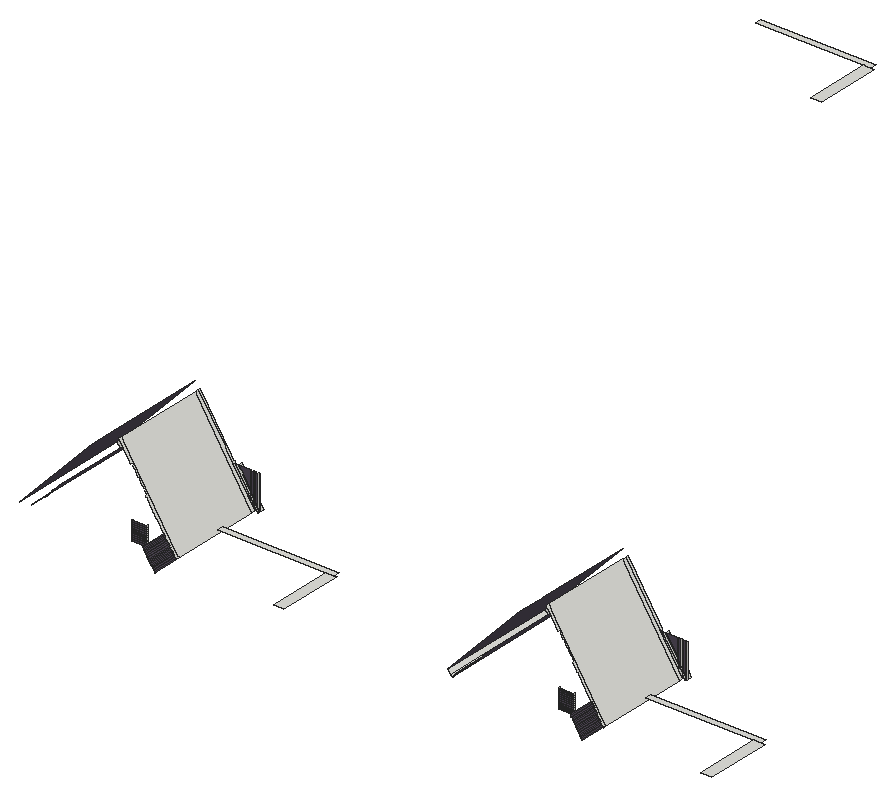
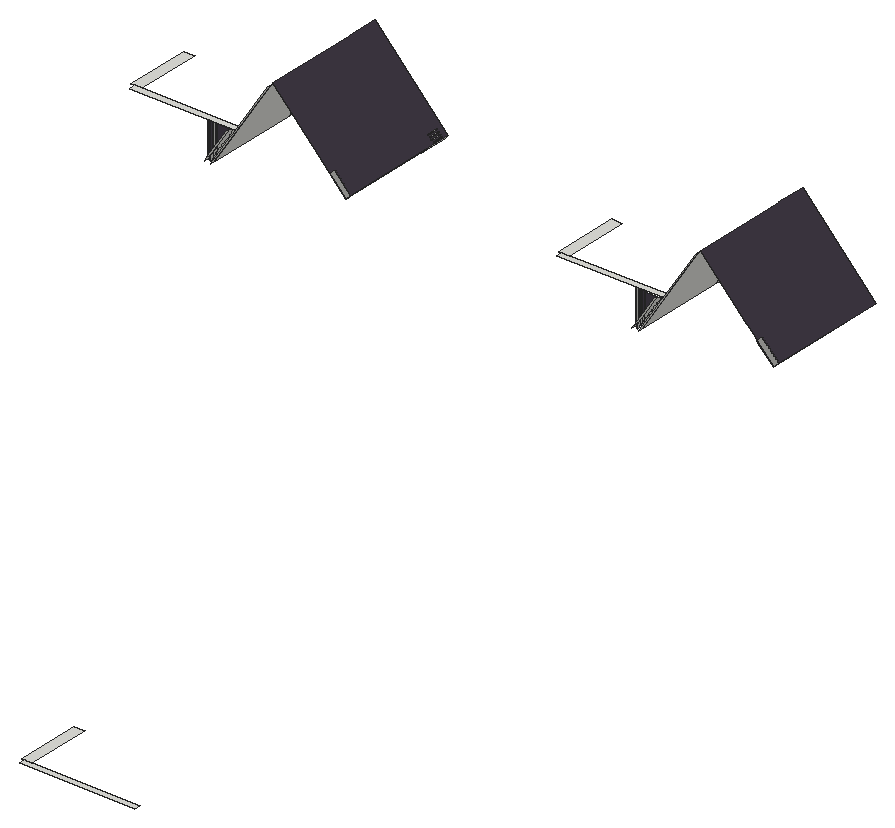
# SketchUp Ruby script. Lengths in inches.
U = 1.inch
M = Sketchup.active_model
def pt(a) = Geom::Point3d.new(a.map { |v| v * U })
def face(e, loops, mat)
  f = e.add_face(loops[0].map { |a| pt(a) })
  loops[1..].each { |l| e.add_face(l.map { |a| pt(a) }).erase! }
  f.material = f.back_material = mat if mat
  f
end
# faces: each face lists its corners as indices into pts; further lists are holes
def faces(e, pts, list, mat = nil) = list.each { |f| face(e, (f[0].is_a?(Array) ? f : [f]).map { |l| l.map { |i| pts[i] } }, mat) }
# xy, xz, yz: faces in a plane at the given z, y or x. An outline is a flat list of corners, or four numbers for a rectangle; further outlines are holes
def ring(l) = l.size == 4 ? [[l[0], l[1]], [l[2], l[1]], [l[2], l[3]], [l[0], l[3]]] : l.each_slice(2).to_a
def flat(e, list, mat, &to3) = list.each { |f| face(e, (f[0].is_a?(Array) ? f : [f]).map { |l| ring(l).map { |u, v| to3.(u, v) } }, mat) }
def xy(e, z, list, mat = nil) = flat(e, list, mat) { |x, y| [x, y, z] }
def xz(e, y, list, mat = nil) = flat(e, list, mat) { |x, z| [x, y, z] }
def yz(e, x, list, mat = nil) = flat(e, list, mat) { |y, z| [x, y, z] }
def lines(e, pts, list) = list.each { |a, b| e.add_line(pt(pts[a]), pt(pts[b])) }
# prism: a flat outline (further loops are holes) pulled along v
def prism(e, loops, v, mat = nil)
  f = face(e, loops, mat); d = Geom::Vector3d.new(v.map { |x| x * U })
  f.pushpull(f.normal.samedirection?(d) ? d.length : -d.length)
end
def box(e, o, s, mat = nil) = prism(e, [[o, [o[0] + s[0], o[1], o[2]], [o[0] + s[0], o[1] + s[1], o[2]], [o[0], o[1] + s[1], o[2]]]], [0, 0, s[2]], mat)
def at(x, y, z, deg = 0) = Geom::Transformation.translation(pt([x, y, z])) * Geom::Transformation.rotation(ORIGIN, Z_AXIS, deg.degrees)
def axes(o, x, y, z) = Geom::Transformation.new([*x, 0, *y, 0, *z, 0, *pt(o).to_a, 1])
def part(name) = M.definitions.add(name)
# library, detail: a bought-in or finely detailed component or shape, given as its bounding box
def library(name, o, s) = part(name).tap { |d| box(d.entities, o, s) }
def detail(e, o, s) = box(e.add_group.entities, o, s)
def put(e, d, t, mat = nil) = e.add_instance(d, t).tap { |i| i.material = mat if mat }
def group(e, t, mat = nil) = e.add_group.tap { |g| g.transformation = t; g.material = mat if mat }.entities
root = M.entities
M.materials.add("[Color M06]").color = [79, 71, 84]
xy(root,267.02,[[1464.52,523.75,1495.49,526.125],[2350.98,523.75,2381.95,526.125]])
xy(root,267.83,[[1464.52,523.75,1495.49,526.125],[2350.98,523.75,2381.95,526.125]])
xy(root,270.95,[[1464.52,523.75,1495.49,526.125],[2350.98,523.75,2381.95,526.125]])
xy(root,271.76,[[1464.52,523.75,1495.49,526.125],[2350.98,523.75,2381.95,526.125]])
xy(root,274.89,[[1464.52,523.75,1495.49,526.125],[2350.98,523.75,2381.95,526.125]])
xy(root,275.7,[[1464.52,523.75,1495.49,526.125],[2350.98,523.75,2381.95,526.125]])
xy(root,278.1875,[[1787.6875,487.3125,1810.23,623.84],[2674.15,487.3125,2696.7,623.84],[1563.99,623.84,1803.23,636.82],[2450.46,623.84,2689.7,636.82],[1419.96,2339.31,1442.5,2475.84],
  [1196.26,2475.84,1435.5,2488.81]])
xy(root,278.83,[[1464.52,523.75,1495.49,526.125],[2350.98,523.75,2381.95,526.125]])
xy(root,279.64,[[1464.52,523.75,1495.49,526.125],[2350.98,523.75,2381.95,526.125]])
xy(root,282.77,[[1464.52,523.75,1495.49,526.125],[2350.98,523.75,2381.95,526.125]])
xy(root,283.58,[[1464.52,523.75,1495.49,526.125],[2350.98,523.75,2381.95,526.125]],"[Color M06]")
xy(root,286.7,[[1464.52,523.75,1495.49,526.125],[2350.98,523.75,2381.95,526.125]])
xy(root,287.51,[[1464.52,523.75,1495.49,526.125],[2350.98,523.75,2381.95,526.125]],"[Color M06]")
xy(root,290.64,[[1464.52,523.75,1495.49,526.125],[2350.98,523.75,2381.95,526.125]])
xy(root,291.45,[[1464.52,523.75,1495.49,526.125],[2350.98,523.75,2381.95,526.125]],"[Color M06]")
xy(root,294.58,[[1464.52,523.75,1495.49,526.125],[2350.98,523.75,2381.95,526.125]])
xy(root,295.39,[[1464.52,523.75,1495.49,526.125],[2350.98,523.75,2381.95,526.125]])
xy(root,298.52,[[1464.52,523.75,1495.49,526.125],[2350.98,523.75,2381.95,526.125]])
xy(root,299.33,[[1464.52,523.75,1495.49,526.125],[2350.98,523.75,2381.95,526.125]])
xy(root,302.45,[[1464.52,523.75,1495.49,526.125],[2350.98,523.75,2381.95,526.125]])
xy(root,303.26,[[1464.52,523.75,1495.49,526.125],[2350.98,523.75,2381.95,526.125]])
xz(root,521.5625,[[1557.92,265.95,1557.66,266.36,1557.92,266.53],[2444.39,265.95,2444.125,266.36,2444.39,266.53],[1557.13,267.19,1557.39,267.36,1555.7,270,1555.43,269.84],[2443.59,267.19,2443.86,267.36,2442.16,270,2441.9,269.84],[1554.9,270.67,1555.16,270.83,1553.47,273.48,1553.21,273.31],
  [2441.37,270.67,2441.63,270.83,2439.93,273.48,2439.67,273.31],[1552.68,274.14,1552.9375,274.31,1551.24,276.95,1550.98,276.78],[2439.14,274.14,2439.4,274.31,2437.71,276.95,2437.44,276.78],[1550.45,277.61,1550.71,277.78,1549.02,280.42,1548.75,280.25],[2436.91,277.61,2437.18,277.78,2435.48,280.42,2435.22,280.25],
  [1548.22,281.08,1548.49,281.25,1546.79,283.89,1546.53,283.73],[2434.6875,281.08,2434.95,281.25,2433.26,283.89,2432.99,283.73],[1546,284.56,1546.26,284.72,1544.56,287.37,1544.3,287.2],[2432.46,284.56,2432.72,284.72,2431.03,287.37,2430.77,287.2],[1543.77,288.03,1544.03,288.2,1542.34,290.84,1542.08,290.67],
  [2430.23,288.03,2430.5,288.2,2428.8,290.84,2428.54,290.67],[1289.04,289.13,1288.59,289.56,1291.01,292.13,1291.46,291.7],[2175.5,289.13,2175.05,289.56,2177.47,292.13,2177.93,291.7],[1541.54,291.5,1539.85,294.14,1540.11,294.3125,1541.81,291.67],[1541.54,291.5,1541.81,291.67,1540.11,294.3125,1539.85,294.14],
  [2428.01,291.5,2426.3125,294.14,2426.58,294.3125,2428.27,291.67],[1292.34,292.64,1291.88,293.0625,1294.3,295.64,1294.76,295.21],[2178.8,292.64,2178.35,293.0625,2180.77,295.64,2181.22,295.21],[1539.32,294.97,1537.62,297.62,1537.89,297.79,1539.58,295.14],[2425.78,294.97,2426.04,295.14,2424.35,297.79,2424.09,297.62],
  [1295.64,296.14,1295.18,296.57,1297.6,299.14,1298.06,298.71],[2182.1,296.14,2181.65,296.57,2184.07,299.14,2184.52,298.71],[1537.09,298.45,1535.4,301.09,1535.66,301.26,1537.35,298.61],[2423.55,298.45,2423.82,298.61,2422.125,301.26,2421.86,301.09],[1298.9375,299.64,1298.48,300.07,1300.9,302.64,1301.36,302.22],
  [2185.4,299.64,2184.94,300.07,2187.37,302.64,2187.82,302.22],[1534.76,301.85,1535.13,302.09,1533.43,304.73,1533.07,304.49],[2421.22,301.85,2421.59,302.09,2419.9,304.73,2419.53,304.49],[1302.23,303.15,1301.78,303.58,1304.2,306.15,1304.66,305.72],[2188.7,303.15,2188.24,303.58,2190.66,306.15,2191.12,305.72],
  [1301.78,303.58,1301.55,303.79,1303.97,306.36,1304.2,306.15],[2188.24,303.58,2188.02,303.79,2190.4375,306.36,2190.66,306.15]])
xz(root,523.75,[[1464.52,267.83,1495.49,270.95],[2350.98,267.83,2381.95,270.95],[1464.52,271.76,1495.49,274.89],[2350.98,271.76,2381.95,274.89],[1464.52,275.7,1495.49,278.83],
  [2350.98,275.7,2381.95,278.83],[1464.52,279.64,1495.49,282.77],[2350.98,279.64,2381.95,282.77],[1464.52,283.58,1495.49,286.7],[2350.98,283.58,2381.95,286.7],
  [1464.52,287.51,1495.49,290.64],[2350.98,287.51,2381.95,290.64],[1464.52,291.45,1495.49,294.58],[2350.98,291.45,2381.95,294.58],[1464.52,295.39,1495.49,298.52],
  [2350.98,295.39,2381.95,298.52],[1464.52,299.33,1495.49,302.45],[2350.98,299.33,2381.95,302.45],[1464.52,303.26,1495.49,306.39],[2350.98,303.26,2381.95,306.39]],"[Color M06]")
xz(root,526.125,[[1464.52,302.45,1495.49,303.26],[2350.98,302.45,2381.95,303.26]])
xz(root,526.125,[[1464.52,267.02,1495.49,267.83],[2350.98,267.02,2381.95,267.83],[1464.52,270.95,1495.49,271.76],[2350.98,270.95,2381.95,271.76],[1464.52,274.89,1495.49,275.7],
  [2350.98,274.89,2381.95,275.7],[1464.52,278.83,1495.49,279.64],[2350.98,278.83,2381.95,279.64],[1464.52,282.77,1495.49,283.58],[2350.98,282.77,2381.95,283.58],
  [1464.52,286.7,1495.49,287.51],[2350.98,286.7,2381.95,287.51],[1464.52,290.64,1495.49,291.45],[2350.98,290.64,2381.95,291.45],[1464.52,294.58,1495.49,295.39],
  [2350.98,294.58,2381.95,295.39],[1464.52,298.52,1495.49,299.33],[2350.98,298.52,2381.95,299.33]],"[Color M06]")
xz(root,719.2,[[1288.59,289.56,1285.45,292.52,1277.91,299.61,1312.29,336.13,1322.96,326.08,1316.04,318.73],[2175.05,289.56,2171.91,292.52,2164.37,299.61,2198.75,336.13,2209.43,326.08,2202.51,318.73]])
xz(root,724.8125,[[1565.73,274.85,1565.73,340.125,1559.65,340.125,1559.65,284.33,1563.99,277.56],[2452.2,274.85,2452.2,340.125,2446.12,340.125,2446.12,284.33,2450.46,277.56],[1556.23,289.67,1556.23,340.125,1550.15,340.125,1550.15,299.15],[2442.7,289.67,2442.7,340.125,2436.62,340.125,2436.62,299.15]],"[Color M06]")
xz(root,726.125,[[1563.99,265.98,1563.99,277.56,1559.65,284.33,1559.65,272.75],[1563.99,265.98,1565.73,267.09,1565.73,274.85,1563.99,277.56],[2450.46,265.98,2450.46,277.56,2446.12,284.33,2446.12,272.75],[2450.46,265.98,2452.2,267.09,2452.2,274.85,2450.46,277.56],[1565.73,267.09,1565.73,274.85,1569.15,269.51,1569.15,269.29],
  [2452.2,267.09,2452.2,274.85,2455.62,269.51,2455.62,269.29],[1556.23,269.17,1556.23,278.09,1550.15,287.57,1550.15,278.65],[2442.7,269.17,2442.7,278.09,2436.62,287.57,2436.62,278.65],[1569.15,269.29,1569.26,269.35,1569.15,269.51],[2455.62,269.29,2455.72,269.35,2455.62,269.51],
  [1559.65,272.75,1559.65,284.33,1556.23,289.67,1556.23,278.09],[2446.12,272.75,2446.12,284.33,2442.7,289.67,2442.7,278.09],[1556.23,278.09,1556.23,289.67,1550.15,299.15,1550.15,287.57],[2442.7,278.09,2442.7,289.67,2436.62,299.15,2436.62,287.57],[1550.15,278.65,1550.15,287.57,1516.46,340.125,1510.74,340.125],
  [2436.62,278.65,2436.62,287.57,2402.92,340.125,2397.21,340.125],[1550.15,287.57,1550.15,299.15,1523.88,340.125,1516.46,340.125],[2436.62,287.57,2436.62,299.15,2410.35,340.125,2402.92,340.125]])
xz(root,726.125,[[1569.15,269.51,1569.15,340.125,1565.73,340.125,1565.73,274.85],[2455.62,269.51,2455.62,340.125,2452.2,340.125,2452.2,274.85],[1559.65,284.33,1559.65,340.125,1556.23,340.125,1556.23,289.67],[2446.12,284.33,2446.12,340.125,2442.7,340.125,2442.7,289.67],[1550.15,299.15,1550.15,340.125,1523.88,340.125],
  [2436.62,299.15,2436.62,340.125,2410.35,340.125]],"[Color M06]")
yz(root,1464.52,[[523.75,267.83,526.125,270.95],[523.75,271.76,526.125,274.89],[523.75,275.7,526.125,278.83],[523.75,279.64,526.125,282.77],[523.75,283.58,526.125,286.7],
  [523.75,287.51,526.125,290.64],[523.75,291.45,526.125,294.58],[523.75,295.39,526.125,298.52],[523.75,299.33,526.125,302.45],[523.75,303.26,526.125,306.39]])
yz(root,1495.49,[[523.75,267.83,526.125,270.95],[523.75,271.76,526.125,274.89],[523.75,275.7,526.125,278.83],[523.75,279.64,526.125,282.77],[523.75,283.58,526.125,286.7],
  [523.75,287.51,526.125,290.64],[523.75,291.45,526.125,294.58],[523.75,295.39,526.125,298.52],[523.75,299.33,526.125,302.45],[523.75,303.26,526.125,306.39]])
yz(root,1550.15,[[724.8125,299.15,726.125,340.125]])
yz(root,1556.23,[[724.8125,289.67,726.125,340.125]])
yz(root,1559.65,[[724.8125,284.33,726.125,340.125]])
yz(root,1565.73,[[724.8125,274.85,726.125,340.125]])
yz(root,1569.15,[[724.8125,269.51,726.125,340.125]])
yz(root,2350.98,[[523.75,267.83,526.125,270.95],[523.75,271.76,526.125,274.89],[523.75,275.7,526.125,278.83],[523.75,279.64,526.125,282.77],[523.75,283.58,526.125,286.7],
  [523.75,287.51,526.125,290.64],[523.75,291.45,526.125,294.58],[523.75,295.39,526.125,298.52],[523.75,299.33,526.125,302.45],[523.75,303.26,526.125,306.39]])
yz(root,2381.95,[[523.75,267.83,526.125,270.95],[523.75,271.76,526.125,274.89],[523.75,275.7,526.125,278.83],[523.75,279.64,526.125,282.77],[523.75,283.58,526.125,286.7],
  [523.75,287.51,526.125,290.64],[523.75,291.45,526.125,294.58],[523.75,295.39,526.125,298.52],[523.75,299.33,526.125,302.45],[523.75,303.26,526.125,306.39]])
yz(root,2436.62,[[724.8125,299.15,726.125,340.125]])
yz(root,2442.7,[[724.8125,289.67,726.125,340.125]])
yz(root,2446.12,[[724.8125,284.33,726.125,340.125]])
yz(root,2452.2,[[724.8125,274.85,726.125,340.125]])
yz(root,2455.62,[[724.8125,269.51,726.125,340.125]])
p = [[1557.92,467.1875,266.53],[1557.92,521.5625,266.53],[1557.66,521.5625,266.36],[1557.66,467.1875,266.36],[2444.39,467.1875,266.53],[2444.39,521.5625,266.53],
  [2444.125,521.5625,266.36],[2444.125,467.1875,266.36],[1557.39,467.1875,267.36],[1557.39,521.5625,267.36],[2443.86,467.1875,267.36],[2443.86,521.5625,267.36],
  [1557.92,528.48,266.53],[1440.02,528.48,450.4375],[1440.02,521.5625,450.4375],[1440.4,521.5625,449.84],[1441.59,521.5625,447.99],[1442.14,521.5625,447.125],
  [1442.59,521.5625,446.42],[1443.78,521.5625,444.57],[1444.34,521.5625,443.7],[1444.79,521.5625,443],[1445.97,521.5625,441.15],[1446.53,521.5625,440.28],
  [1446.98,521.5625,439.58],[1448.17,521.5625,437.73],[1448.72,521.5625,436.86],[1449.17,521.5625,436.16],[1450.36,521.5625,434.31],[1450.91,521.5625,433.44],
  [1451.36,521.5625,432.74],[1452.55,521.5625,430.89],[1453.11,521.5625,430.02],[1453.56,521.5625,429.32],[1454.74,521.5625,427.47],[1455.3,521.5625,426.6],
  [1455.75,521.5625,425.9],[1456.9375,521.5625,424.05],[1457.49,521.5625,423.18],[1457.94,521.5625,422.48],[1459.13,521.5625,420.63],[1459.68,521.5625,419.76],
  [1460.13,521.5625,419.0625],[1461.32,521.5625,417.21],[1461.875,521.5625,416.34],[1462.33,521.5625,415.64],[1463.51,521.5625,413.79],[1464.07,521.5625,412.92],
  [1464.52,521.5625,412.22],[1464.52,526.125,412.22],[1464.58,526.125,412.12],[1466.59,526.125,409],[1467.47,526.125,407.62],[1467.47,524.25,407.62],
  [1469.47,524.25,404.5],[1469.47,526.125,404.5],[1470.19,526.125,403.37],[1470.19,524.25,403.37],[1472.2,524.25,400.25],[1472.2,526.125,400.25],
  [1472.92,526.125,399.12],[1472.92,524.25,399.12],[1474.92,524.25,396],[1474.92,526.125,396],[1475.64,526.125,394.87],[1475.64,524.25,394.87],
  [1477.65,524.25,391.75],[1477.65,526.125,391.75],[1478.37,526.125,390.62],[1478.37,524.25,390.62],[1480.37,524.25,387.5],[1480.37,526.125,387.5],
  [1481.09,526.125,386.37],[1481.09,524.25,386.37],[1483.1,524.25,383.25],[1483.1,526.125,383.25],[1483.82,526.125,382.12],[1483.82,524.25,382.12],
  [1485.82,524.25,379],[1485.82,526.125,379],[1486.54,526.125,377.87],[1486.54,524.25,377.87],[1488.55,524.25,374.75],[1488.55,526.125,374.75],
  [1489.27,526.125,373.62],[1491.27,526.125,370.5],[1491.99,526.125,369.37],[1491.99,524.25,369.37],[1494,524.25,366.25],[1494,526.125,366.25],
  [1494.72,526.125,365.12],[1495.49,526.125,363.92],[1495.49,524.25,363.92],[1495.49,521.5625,363.92],[1496.67,521.5625,362.07],[1497.31,521.5625,361.08],
  [1497.36,521.5625,360.99],[1499,521.5625,358.4375],[1499.63,521.5625,357.45],[1501.33,521.5625,354.81],[1501.96,521.5625,353.82],[1503.66,521.5625,351.18],
  [1504.29,521.5625,350.19],[1505.98,521.5625,347.55],[1506.62,521.5625,346.56],[1508.3125,521.5625,343.92],[1508.94,521.5625,342.93],[1510.64,521.5625,340.29],
  [1510.74,521.5625,340.125],[1511.17,521.5625,339.46],[1512.86,521.5625,336.8125],[1513.4,521.5625,335.98],[1515.09,521.5625,333.34],[1515.62,521.5625,332.51],
  [1517.32,521.5625,329.87],[1517.85,521.5625,329.04],[1519.54,521.5625,326.4],[1520.08,521.5625,325.57],[1521.77,521.5625,322.92],[1522.3,521.5625,322.09],
  [1524,521.5625,319.45],[1524.53,521.5625,318.62],[1526.22,521.5625,315.98],[1526.75,521.5625,315.15],[1528.45,521.5625,312.51],[1528.98,521.5625,311.68],
  [1530.68,521.5625,309.03],[1531.21,521.5625,308.2],[1532.9,521.5625,305.56],[1533.43,521.5625,304.73],[1535.13,521.5625,302.09],[1535.66,521.5625,301.26],
  [1537.35,521.5625,298.61],[1537.89,521.5625,297.79],[1539.58,521.5625,295.14],[1540.11,521.5625,294.3125],[1541.81,521.5625,291.67],[1542.34,521.5625,290.84],
  [1544.03,521.5625,288.2],[1544.56,521.5625,287.37],[1546.26,521.5625,284.72],[1546.79,521.5625,283.89],[1548.49,521.5625,281.25],[1549.02,521.5625,280.42],
  [1550.71,521.5625,277.78],[1551.24,521.5625,276.95],[1552.9375,521.5625,274.31],[1553.47,521.5625,273.48],[1555.16,521.5625,270.83],[1555.7,521.5625,270],
  [2444.39,528.48,266.53],[2326.48,528.48,450.4375],[2326.48,521.5625,450.4375],[2326.86,521.5625,449.84],[2328.05,521.5625,447.99],[2328.61,521.5625,447.125],
  [2329.06,521.5625,446.42],[2330.24,521.5625,444.57],[2330.8,521.5625,443.7],[2331.25,521.5625,443],[2332.4375,521.5625,441.15],[2332.99,521.5625,440.28],
  [2333.44,521.5625,439.58],[2334.63,521.5625,437.73],[2335.18,521.5625,436.86],[2335.63,521.5625,436.16],[2336.82,521.5625,434.31],[2337.38,521.5625,433.44],
  [2337.83,521.5625,432.74],[2339.02,521.5625,430.89],[2339.57,521.5625,430.02],[2340.02,521.5625,429.32],[2341.21,521.5625,427.47],[2341.76,521.5625,426.6],
  [2342.21,521.5625,425.9],[2343.4,521.5625,424.05],[2343.96,521.5625,423.18],[2344.41,521.5625,422.48],[2345.59,521.5625,420.63],[2346.15,521.5625,419.76],
  [2346.6,521.5625,419.0625],[2347.79,521.5625,417.21],[2348.34,521.5625,416.34],[2348.79,521.5625,415.64],[2349.98,521.5625,413.79],[2350.53,521.5625,412.92],
  [2350.98,521.5625,412.22],[2350.98,526.125,412.22],[2351.05,526.125,412.12],[2353.05,526.125,409],[2353.93,526.125,407.62],[2353.93,524.25,407.62],
  [2355.9375,524.25,404.5],[2355.9375,526.125,404.5],[2356.66,526.125,403.37],[2356.66,524.25,403.37],[2358.66,524.25,400.25],[2358.66,526.125,400.25],
  [2359.38,526.125,399.12],[2359.38,524.25,399.12],[2361.39,524.25,396],[2361.39,526.125,396],[2362.11,526.125,394.87],[2362.11,524.25,394.87],
  [2364.11,524.25,391.75],[2364.11,526.125,391.75],[2364.83,526.125,390.62],[2364.83,524.25,390.62],[2366.84,524.25,387.5],[2366.84,526.125,387.5],
  [2367.56,526.125,386.37],[2367.56,524.25,386.37],[2369.5625,524.25,383.25],[2369.5625,526.125,383.25],[2370.28,526.125,382.12],[2370.28,524.25,382.12],
  [2372.29,524.25,379],[2372.29,526.125,379],[2373.01,526.125,377.87],[2373.01,524.25,377.87],[2375.01,524.25,374.75],[2375.01,526.125,374.75],
  [2375.73,526.125,373.62],[2377.73,526.125,370.5],[2378.45,526.125,369.37],[2378.45,524.25,369.37],[2380.46,524.25,366.25],[2380.46,526.125,366.25],
  [2381.18,526.125,365.12],[2381.95,526.125,363.92],[2381.95,524.25,363.92],[2381.95,521.5625,363.92],[2383.14,521.5625,362.07],[2383.77,521.5625,361.08],
  [2383.83,521.5625,360.99],[2385.46,521.5625,358.4375],[2386.1,521.5625,357.45],[2387.79,521.5625,354.81],[2388.43,521.5625,353.82],[2390.12,521.5625,351.18],
  [2390.75,521.5625,350.19],[2392.45,521.5625,347.55],[2393.08,521.5625,346.56],[2394.77,521.5625,343.92],[2395.41,521.5625,342.93],[2397.1,521.5625,340.29],
  [2397.21,521.5625,340.125],[2397.63,521.5625,339.46],[2399.33,521.5625,336.8125],[2399.86,521.5625,335.98],[2401.55,521.5625,333.34],[2402.09,521.5625,332.51],
  [2403.78,521.5625,329.87],[2404.3125,521.5625,329.04],[2406.01,521.5625,326.4],[2406.54,521.5625,325.57],[2408.23,521.5625,322.92],[2408.77,521.5625,322.09],
  [2410.46,521.5625,319.45],[2410.99,521.5625,318.62],[2412.6875,521.5625,315.98],[2413.22,521.5625,315.15],[2414.91,521.5625,312.51],[2415.44,521.5625,311.68],
  [2417.14,521.5625,309.03],[2417.67,521.5625,308.2],[2419.37,521.5625,305.56],[2419.9,521.5625,304.73],[2421.59,521.5625,302.09],[2422.125,521.5625,301.26],
  [2423.82,521.5625,298.61],[2424.35,521.5625,297.79],[2426.04,521.5625,295.14],[2426.58,521.5625,294.3125],[2428.27,521.5625,291.67],[2428.8,521.5625,290.84],
  [2430.5,521.5625,288.2],[2431.03,521.5625,287.37],[2432.72,521.5625,284.72],[2433.26,521.5625,283.89],[2434.95,521.5625,281.25],[2435.48,521.5625,280.42],
  [2437.18,521.5625,277.78],[2437.71,521.5625,276.95],[2439.4,521.5625,274.31],[2439.93,521.5625,273.48],[2441.63,521.5625,270.83],[2442.16,521.5625,270],
  [1557.92,719.59,266.53],[1440.02,719.59,450.4375],[2444.39,719.59,266.53],[2326.48,719.59,450.4375],[1510.74,726.125,340.125],[1550.15,726.125,278.65],
  [1556.23,726.125,269.17],[1557.92,726.125,266.53],[1440.02,726.125,450.4375],[1494.83,726.125,364.9375],[1497.82,726.125,360.28],[1504.29,726.125,350.1875],
  [2397.21,726.125,340.125],[2436.62,726.125,278.65],[2442.7,726.125,269.17],[2444.39,726.125,266.53],[2326.48,726.125,450.4375],[2381.3,726.125,364.9375],
  [2384.28,726.125,360.28],[2390.75,726.125,350.1875],[1440.02,731.75,450.4375],[1557.92,732.2,266.53],[1518.52,732.2,328],[1517.43,732.2,329.69],
  [1511.54,732.2,338.875],[1510.74,732.2,340.125],[1510.01,732.2,341.27],[1504.29,732.2,350.1875],[1440.02,732.2,450.4375],[2326.48,731.75,450.4375],
  [2444.39,732.2,266.53],[2404.98,732.2,328],[2403.9,732.2,329.69],[2398.01,732.2,338.875],[2397.21,732.2,340.125],[2396.47,732.2,341.27],
  [2390.75,732.2,350.1875],[2326.48,732.2,450.4375],[1555.43,521.5625,269.84],[1557.13,521.5625,267.19],[1557.13,467.1875,267.19],[1555.43,467.1875,269.84],
  [2441.9,521.5625,269.84],[2443.59,521.5625,267.19],[2443.59,467.1875,267.19],[2441.9,467.1875,269.84],[1569.26,726.125,269.35],[1569.15,726.125,269.51],
  [1569.15,724.8125,269.51],[1569.26,724.8125,269.35],[2455.72,726.125,269.35],[2455.62,726.125,269.51],[2455.62,724.8125,269.51],[2455.72,724.8125,269.35],
  [1565.73,726.125,274.85],[1563.99,726.125,277.56],[1563.99,734.4375,277.56],[1569.26,734.4375,269.35],[2452.2,726.125,274.85],[2450.46,726.125,277.56],
  [2450.46,734.4375,277.56],[2455.72,734.4375,269.35],[1555.7,467.1875,270],[2442.16,467.1875,270],[1555.16,467.1875,270.83],[2441.63,467.1875,270.83],
  [1553.21,521.5625,273.31],[1554.9,521.5625,270.67],[1554.9,467.1875,270.67],[1553.21,467.1875,273.31],[2439.67,521.5625,273.31],[2441.37,521.5625,270.67],
  [2441.37,467.1875,270.67],[2439.67,467.1875,273.31],[1553.47,467.1875,273.48],[2439.93,467.1875,273.48],[1552.9375,467.1875,274.31],[2439.4,467.1875,274.31],
  [1550.98,521.5625,276.78],[1552.68,521.5625,274.14],[1552.68,467.1875,274.14],[1550.98,467.1875,276.78],[2437.44,521.5625,276.78],[2439.14,521.5625,274.14],
  [2439.14,467.1875,274.14],[2437.44,467.1875,276.78],[1563.99,724.8125,277.56],[1565.73,724.8125,274.85],[2450.46,724.8125,277.56],[2452.2,724.8125,274.85],
  [1551.24,467.1875,276.95],[2437.71,467.1875,276.95],[1550.71,467.1875,277.78],[2437.18,467.1875,277.78],[1548.75,521.5625,280.25],[1550.45,521.5625,277.61],
  [1550.45,467.1875,277.61],[1548.75,467.1875,280.25],[2435.22,521.5625,280.25],[2436.91,521.5625,277.61],[2436.91,467.1875,277.61],[2435.22,467.1875,280.25],
  [1559.65,726.125,284.33],[1559.65,724.8125,284.33],[2446.12,726.125,284.33],[2446.12,724.8125,284.33],[1550.15,726.125,299.15],[1523.88,726.125,340.125],
  [1523.88,732.2,340.125],[1523.88,734.4375,340.125],[1556.23,726.125,289.67],[2436.62,726.125,299.15],[2410.35,726.125,340.125],[2410.35,732.2,340.125],
  [2410.35,734.4375,340.125],[2442.7,726.125,289.67],[1549.02,467.1875,280.42],[2435.48,467.1875,280.42],[1548.49,467.1875,281.25],[2434.95,467.1875,281.25],
  [1546.53,521.5625,283.73],[1548.22,521.5625,281.08],[1548.22,467.1875,281.08],[1546.53,467.1875,283.73],[2432.99,521.5625,283.73],[2434.6875,521.5625,281.08],
  [2434.6875,467.1875,281.08],[2432.99,467.1875,283.73],[1546.79,467.1875,283.89],[2433.26,467.1875,283.89],[1546.26,467.1875,284.72],[2432.72,467.1875,284.72],
  [1544.3,521.5625,287.2],[1546,521.5625,284.56],[1546,467.1875,284.56],[1544.3,467.1875,287.2],[2430.77,521.5625,287.2],[2432.46,521.5625,284.56],
  [2432.46,467.1875,284.56],[2430.77,467.1875,287.2],[1544.56,467.1875,287.37],[2431.03,467.1875,287.37],[1544.03,467.1875,288.2],[2430.5,467.1875,288.2],
  [1542.08,521.5625,290.67],[1543.77,521.5625,288.03],[1543.77,467.1875,288.03],[1542.08,467.1875,290.67],[2428.54,521.5625,290.67],[2430.23,521.5625,288.03],
  [2430.23,467.1875,288.03],[2428.54,467.1875,290.67],[2175.05,467.1875,289.56],[2175.05,521.5625,289.56],[2175.5,521.5625,289.13],[2175.5,467.1875,289.13],
  [2177.93,521.5625,291.7],[2177.93,467.1875,291.7],[2171.91,467.1875,292.52],[2171.91,528.48,292.52],[2171.91,719.2,292.52],[2175.05,719.2,289.56],
  [2177.47,521.5625,292.13],[2177.47,467.1875,292.13],[1322.96,719.2,326.08],[1322.96,528.48,326.08],[1322.96,521.5625,326.08],[1321.57,521.5625,324.6],
  [1320.69,521.5625,323.67],[1318.27,521.5625,321.1],[1317.39,521.5625,320.17],[1316.04,521.5625,318.73],[1314.97,521.5625,317.59],[1314.1,521.5625,316.66],
  [1311.68,521.5625,314.09],[1310.8,521.5625,313.16],[1308.375,521.5625,310.59],[1307.5,521.5625,309.65],[1305.08,521.5625,307.08],[1304.2,521.5625,306.15],
  [1301.78,521.5625,303.58],[1300.9,521.5625,302.64],[1298.48,521.5625,300.07],[1297.6,521.5625,299.14],[1295.18,521.5625,296.57],[1294.3,521.5625,295.64],
  [1291.88,521.5625,293.0625],[1291.01,521.5625,292.13],[1288.59,521.5625,289.56],[1288.59,719.2,289.56],[1316.04,719.2,318.73],[2209.43,719.2,326.08],
  [2209.43,528.48,326.08],[2209.43,521.5625,326.08],[2208.03,521.5625,324.6],[2207.16,521.5625,323.67],[2204.74,521.5625,321.1],[2203.86,521.5625,320.17],
  [2202.51,521.5625,318.73],[2201.4375,521.5625,317.59],[2200.56,521.5625,316.66],[2198.14,521.5625,314.09],[2197.26,521.5625,313.16],[2194.84,521.5625,310.59],
  [2193.96,521.5625,309.65],[2191.54,521.5625,307.08],[2190.66,521.5625,306.15],[2188.24,521.5625,303.58],[2187.37,521.5625,302.64],[2184.94,521.5625,300.07],
  [2184.07,521.5625,299.14],[2181.65,521.5625,296.57],[2180.77,521.5625,295.64],[2178.35,521.5625,293.0625],[2202.51,719.2,318.73],[1550.15,724.8125,299.15],
  [1556.23,724.8125,289.67],[2436.62,724.8125,299.15],[2442.7,724.8125,289.67],[1542.34,467.1875,290.84],[2428.8,467.1875,290.84],[1541.81,467.1875,291.67],
  [2428.27,467.1875,291.67],[1539.85,521.5625,294.14],[1541.54,521.5625,291.5],[1541.54,467.1875,291.5],[1539.85,467.1875,294.14],[2426.3125,521.5625,294.14],
  [2428.01,521.5625,291.5],[2428.01,467.1875,291.5],[2426.3125,467.1875,294.14],[2178.35,467.1875,293.0625],[2164.37,467.1875,299.61],[2164.37,719.2,299.61],
  [2178.8,521.5625,292.64],[2178.8,467.1875,292.64],[2181.22,521.5625,295.21],[2181.22,467.1875,295.21],[2180.77,467.1875,295.64],[1540.11,467.1875,294.3125],
  [2426.58,467.1875,294.3125],[1539.58,467.1875,295.14],[2426.04,467.1875,295.14],[1537.62,521.5625,297.62],[1539.32,521.5625,294.97],[1539.32,467.1875,294.97],
  [1537.62,467.1875,297.62],[2424.09,521.5625,297.62],[2425.78,521.5625,294.97],[2425.78,467.1875,294.97],[2424.09,467.1875,297.62],[2181.65,467.1875,296.57],
  [2182.1,521.5625,296.14],[2182.1,467.1875,296.14],[2184.52,521.5625,298.71],[2184.52,467.1875,298.71],[2184.07,467.1875,299.14],[1537.89,467.1875,297.79],
  [2424.35,467.1875,297.79],[1537.35,467.1875,298.61],[2423.82,467.1875,298.61],[1535.4,521.5625,301.09],[1537.09,521.5625,298.45],[1537.09,467.1875,298.45],
  [1535.4,467.1875,301.09],[2421.86,521.5625,301.09],[2423.55,521.5625,298.45],[2423.55,467.1875,298.45],[2421.86,467.1875,301.09],[2184.94,467.1875,300.07],
  [1277.91,719.2,299.61],[1277.91,467.1875,299.61],[1430.11,467.1875,461.31],[1430.11,528.48,461.31],[1429.34,528.48,460.49],[1429.34,731.75,460.49],
  [1333.34,731.75,358.5],[1332.61,731.75,357.73],[1316.04,731.75,340.125],[1312.29,731.75,336.13],[1312.29,719.2,336.13],[2316.58,467.1875,461.31],
  [2316.58,528.48,461.31],[2315.81,528.48,460.49],[2315.81,731.75,460.49],[2219.8,731.75,358.5],[2219.08,731.75,357.73],[2202.51,731.75,340.125],
  [2198.75,731.75,336.13],[2198.75,719.2,336.13],[2185.4,521.5625,299.64],[2185.4,467.1875,299.64],[2187.82,521.5625,302.22],[2187.82,467.1875,302.22],
  [2187.37,467.1875,302.64],[1535.66,467.1875,301.26],[2422.125,467.1875,301.26],[1535.13,467.1875,302.09],[2421.59,467.1875,302.09],[1533.07,521.5625,304.49],
  [1534.76,521.5625,301.85],[1534.76,467.1875,301.85],[1533.07,467.1875,304.49],[2419.53,521.5625,304.49],[2421.22,521.5625,301.85],[2421.22,467.1875,301.85],
  [2419.53,467.1875,304.49],[2188.24,467.1875,303.58],[1302.23,521.5625,303.15],[1304.66,521.5625,305.72],[1304.66,467.1875,305.72],[1302.23,467.1875,303.15],
  [2188.7,521.5625,303.15],[2188.7,467.1875,303.15],[2191.12,521.5625,305.72],[2191.12,467.1875,305.72],[2188.02,467.1875,303.79],[2188.02,521.5625,303.79],
  [2190.66,467.1875,306.15],[2190.4375,521.5625,306.36],[2190.4375,467.1875,306.36],[1533.43,467.1875,304.73],[2419.9,467.1875,304.73],[1532.9,467.1875,305.56],
  [2419.37,467.1875,305.56],[1312.9,719.2,321.6875],[1285.45,719.2,292.52],[2199.37,719.2,321.6875]]
faces(root,p,[[0,1,2,3],[4,5,6,7],[12,13,14,15,16,17,18,19,20,21,22,23,24,25,26,27,28,29,30,31,32,33,34,35,36,37,38,39,40,41,42,43,44,45,46,47,48,49,50,51,52,53,54,55,56,57,58,59,60,61,62,63,64,65,66,67,68,69,70,71,72,73,74,75,76,77,78,79,80,81,82,83,84,85,86,87,88,89,90,91,92,93,94,95,96,97,98,99,100,101,102,103,104,105,106,107,108,109,110,111,112,113,114,115,116,117,118,119,120,121,122,123,124,125,126,127,128,129,130,131,132,133,134,135,136,137,138,139,140,141,142,143,144,145,146,147,148,149,9,1],[150,151,152,153,154,155,156,157,158,159,160,161,162,163,164,165,166,167,168,169,170,171,172,173,174,175,176,177,178,179,180,181,182,183,184,185,186,187,188,189,190,191,192,193,194,195,196,197,198,199,200,201,202,203,204,205,206,207,208,209,210,211,212,213,214,215,216,217,218,219,220,221,222,223,224,225,226,227,228,229,230,231,232,233,234,235,236,237,238,239,240,241,242,243,244,245,246,247,248,249,250,251,252,253,254,255,256,257,258,259,260,261,262,263,264,265,266,267,268,269,270,271,272,273,274,275,276,277,278,279,280,281,282,283,284,285,286,287,11,5],[288,12,13,289],[290,150,151,291],[292,293,294,295,288,289,296,297,298,299],[300,301,302,303,290,291,304,305,306,307],
  [308,296,297,298,299,292,293,294,295,309,310,311,312,313,314,315,316],[317,304,305,306,307,300,301,302,303,318,319,320,321,322,323,324,325],[9,8,328,327],[11,10,332,331],[334,335,336,337],[338,339,340,341],[342,343,344,345,334,335],[346,347,348,349,338,339],
  [350,149,326,329],[351,287,330,333],[148,352,356,355],[286,353,360,359],[362,147,354,357],[363,285,358,361],[146,364,368,367],[284,365,372,371],
  [342,343,374,375],[346,347,376,377],[378,145,366,369],[379,283,370,373],[144,380,384,383],[282,381,388,387],[343,390,391,374],[347,392,393,376],
  [394,395,396,397,344,343,390,398],[399,400,401,402,348,347,392,403],[404,143,382,385],[405,281,386,389],[142,406,410,409],[280,407,414,413],[416,141,408,411],[417,279,412,415],
  [140,418,422,421],[278,419,426,425],[428,139,420,423],[429,277,424,427],[138,430,434,433],[276,431,438,437],[440,441,442,443],[440,446,447,448,449,441],
  [450,441,440,451],[398,394,503,504],[403,399,505,506],[507,137,432,435],[508,275,436,439],[136,509,513,512],[274,510,517,516],[450,451,445,444],
  [446,520,521,448,447],[519,501,522,523],[500,501,519,526],[527,135,511,514],[528,273,515,518],[134,529,533,532],[272,530,537,536],[500,526,525,524],
  [539,499,540,541],[498,499,539,544],[545,133,531,534],[546,271,535,538],[132,547,551,550],[270,548,555,554],[498,544,543,542],[557,497,578,579],
  [496,497,557,582],[583,131,549,552],[584,269,553,556],[130,585,589,588],[268,586,593,592],[496,582,581,580],[495,595,604,605],[494,495,595,606],
  [607,605,604,608],[609,129,587,590],[610,267,591,594]])
faces(root,p,[[0,8,9,1],[4,10,11,5],[326,327,328,329],[330,331,332,333],[350,352,148,149],[351,353,286,287],[354,355,356,357],[358,359,360,361],
  [362,364,146,147],[363,365,284,285],[366,367,368,369],[370,371,372,373],[378,380,144,145],[379,381,282,283],[382,383,384,385],[386,387,388,389],
  [404,406,142,143],[405,407,280,281],[408,409,410,411],[412,413,414,415],[416,418,140,141],[417,419,278,279],[420,421,422,423],[424,425,426,427],
  [428,430,138,139],[429,431,276,277],[432,433,434,435],[436,437,438,439],[442,444,445,443],[452,453,454,455,456,457,458,459,460,461,462,463,464,465,466,467,468,469,470,471,472,473,474,475,476,477,478],[479,480,481,482,483,484,485,486,487,488,489,490,491,492,493,494,495,496,497,498,499,500,501,450,441,449,502],[507,509,136,137],
  [508,510,274,275],[511,512,513,514],[515,516,517,518],[450,501,519,451],[522,524,525,523],[527,529,134,135],[528,530,272,273],[531,532,533,534],
  [535,536,537,538],[500,499,539,526],[540,542,543,541],[545,547,132,133],[546,548,270,271],[549,550,551,552],[553,554,555,556],[498,497,557,544],
  [558,559,560,561,562,563,564,565,566,567,568],[521,520,569,570,571,572,573,574,575,576,577],[578,580,581,579],[583,585,130,131],[584,586,268,269],[587,588,589,590],[591,592,593,594],[496,495,595,582],
  [596,597,598,599],[595,495,600,601],[600,602,603,601],[609,611,128,129],[610,612,266,267]],"[Color M06]")
lines(root,p,[[613,614],[615,448]])
